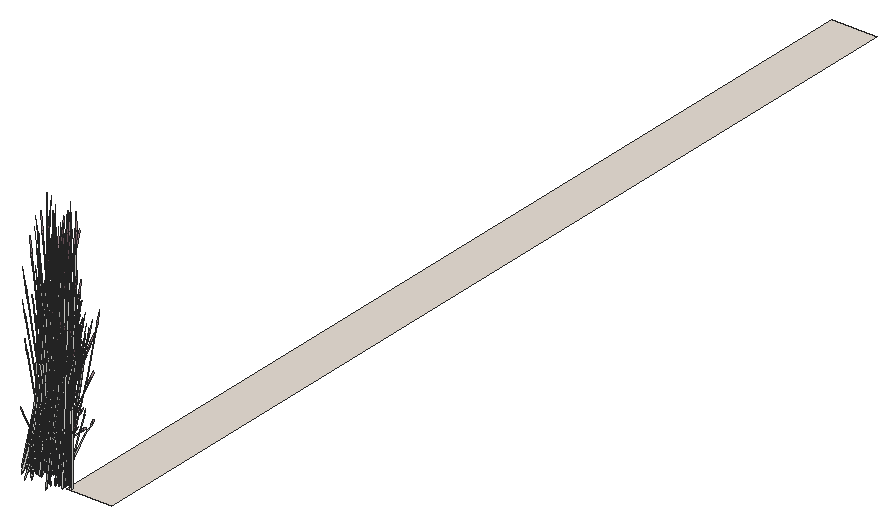
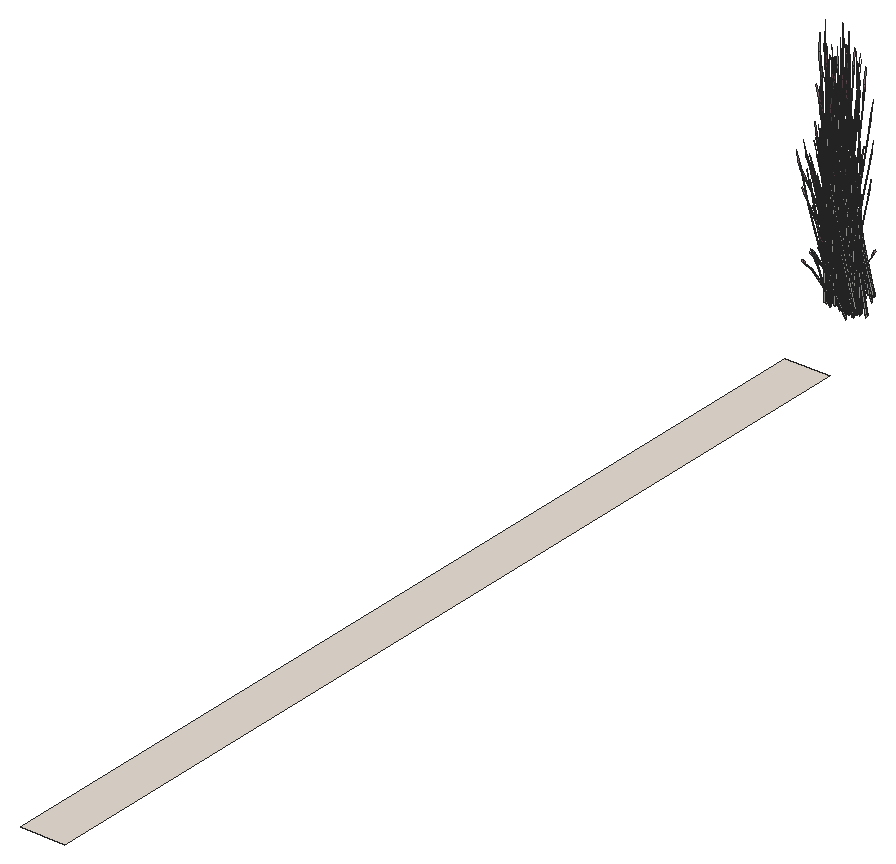
# SketchUp Ruby script. Lengths in inches.
U = 1.inch
M = Sketchup.active_model
def pt(a) = Geom::Point3d.new(a.map { |v| v * U })
def face(e, loops, mat)
  f = e.add_face(loops[0].map { |a| pt(a) })
  loops[1..].each { |l| e.add_face(l.map { |a| pt(a) }).erase! }
  f.material = f.back_material = mat if mat
  f
end
# faces: each face lists its corners as indices into pts; further lists are holes
def faces(e, pts, list, mat = nil) = list.each { |f| face(e, (f[0].is_a?(Array) ? f : [f]).map { |l| l.map { |i| pts[i] } }, mat) }
# xy, xz, yz: faces in a plane at the given z, y or x. An outline is a flat list of corners, or four numbers for a rectangle; further outlines are holes
def ring(l) = l.size == 4 ? [[l[0], l[1]], [l[2], l[1]], [l[2], l[3]], [l[0], l[3]]] : l.each_slice(2).to_a
def flat(e, list, mat, &to3) = list.each { |f| face(e, (f[0].is_a?(Array) ? f : [f]).map { |l| ring(l).map { |u, v| to3.(u, v) } }, mat) }
def xy(e, z, list, mat = nil) = flat(e, list, mat) { |x, y| [x, y, z] }
def xz(e, y, list, mat = nil) = flat(e, list, mat) { |x, z| [x, y, z] }
def yz(e, x, list, mat = nil) = flat(e, list, mat) { |y, z| [x, y, z] }
def lines(e, pts, list) = list.each { |a, b| e.add_line(pt(pts[a]), pt(pts[b])) }
# prism: a flat outline (further loops are holes) pulled along v
def prism(e, loops, v, mat = nil)
  f = face(e, loops, mat); d = Geom::Vector3d.new(v.map { |x| x * U })
  f.pushpull(f.normal.samedirection?(d) ? d.length : -d.length)
end
def box(e, o, s, mat = nil) = prism(e, [[o, [o[0] + s[0], o[1], o[2]], [o[0] + s[0], o[1] + s[1], o[2]], [o[0], o[1] + s[1], o[2]]]], [0, 0, s[2]], mat)
def at(x, y, z, deg = 0) = Geom::Transformation.translation(pt([x, y, z])) * Geom::Transformation.rotation(ORIGIN, Z_AXIS, deg.degrees)
def axes(o, x, y, z) = Geom::Transformation.new([*x, 0, *y, 0, *z, 0, *pt(o).to_a, 1])
def part(name) = M.definitions.add(name)
# library, detail: a bought-in or finely detailed component or shape, given as its bounding box
def library(name, o, s) = part(name).tap { |d| box(d.entities, o, s) }
def detail(e, o, s) = box(e.add_group.entities, o, s)
def put(e, d, t, mat = nil) = e.add_instance(d, t).tap { |i| i.material = mat if mat }
def group(e, t, mat = nil) = e.add_group.tap { |g| g.transformation = t; g.material = mat if mat }.entities
root = M.entities
M.materials.add("LightPink_Translucent").color = [144, 107, 117]
M.materials["LightPink_Translucent"].alpha = 0.75
M.materials.add("Marble_01_1K").color = [230, 221, 211]
c1 = part("blade")
p = [[2.15,0.21,22],[0,0.17,0],[0.09,0.45,0],[2.18,0.31,22],[2.29,0.31,22],[0.38,0.45,0],
  [2.48,0.24,33],[2.49,0.24,33],[2.48,0.22,33]]
faces(c1.entities,p,[[0,1,2,3],[4,5,2,3],[6,3,4,7],[8,0,3,6]])
c2 = part("seeds")
p = [[0.3,-0.1,1.38],[-0.01,-0.03,1.59],[-0.01,-0.03,0.03],[0.14,-0.07,-0.07],[0.29,-0.03,3],[0.15,0.01,3.11]]
faces(c2.entities,p,[[0,1,2,3],[1,0,4,5]],"LightPink_Translucent")
c3 = part("blade with seeds")
put(c3.entities,c1,at(0,0,0))
put(c3.entities,c2,axes([2.4,0.25,30.99],[1.5799,-0.05474,1.17369],[-0.12525,1.92788,0.29478],[-0.07173,-0.02425,1.56792]))
xy(root,36,[[314,46,324,262]],"Marble_01_1K")
put(root,c3,axes([315.7,32.58,46.14],[0.49824,-0.09289,-0.45151],[0.08716,0.35177,-0.34973],[0.13382,0.10081,0.86392]))
put(root,c3,axes([317.83,36.3125,46.16],[-0.06595,-0.00297,1.56736],[-0.27386,-0.31799,-0.1481],[0.10998,-0.10455,0.27737]))
put(root,c3,axes([320.91,35.45,43.82],[-0.52523,-0.06406,-0.55095],[0.11084,-0.39517,-0.1446],[-0.15674,-0.04788,1.21613]))
put(root,c3,axes([314.6,36.14,43.82],[0.34009,-0.2937,-0.55095],[0.42248,0.26632,-0.1446],[0.13628,-0.07327,1.21613]))
put(root,c3,axes([317.05,35.44,44.44],[-0.16818,0.19891,1.01491],[-0.14456,-0.26725,0.74569],[0.1389,-0.06697,0.22354]))
put(root,c3,axes([321.16,30.84,44.97],[0.01109,-0.20172,1.3638],[0.49896,0.10655,0.18846],[-0.04323,0.21498,0.64398]))
put(root,c3,axes([322.19,35.24,44.03],[-0.46965,-0.33633,-0.05417],[0.46994,-0.33653,0],[-0.0164,-0.01174,1.55135]))
put(root,c3,axes([321.01,34.03,44.1875],[-0.14586,0.38834,0.15589],[-0.53375,-0.1099,0.31002],[0.0922,-0.00189,1.41735]))
put(root,c3,axes([316.39,32.93,44.36],[-0.32378,-0.01225,0.92831],[0.21383,-0.26028,0.51254],[0.12791,0.09247,0.72818]))
put(root,c3,axes([319.27,34.71,46.18],[0.14265,-0.35629,0.42415],[0.46898,0.12183,0.34973],[-0.18443,0.02141,0.87768]))
put(root,c3,axes([316.8125,36.1875,46],[0.43951,-0.05584,-0.31292],[0.11606,0.31924,0.40398],[0.12595,-0.08575,0.77298]))
put(root,c3,axes([315.46,32.86,46.18],[-0.22948,0.24822,0.05682],[-0.32679,-0.14452,0.44729],[0.10565,0.07958,0.68204]))
put(root,c3,axes([319.23,34.61,46.18],[-0.18545,-0.26643,0.05682],[0.33817,-0.13041,0.44729],[-0.14907,0.02573,0.68204]))
put(root,c3,axes([321.3,35.29,44.09],[0.63817,0.08233,0.40429],[-0.12987,0.46497,0.15865],[-0.09326,-0.0449,1.40366]))
put(root,c3,axes([314.92,33.7,46.99],[0.34892,-0.22417,-0.05733],[0.3197,0.24551,-0.25992],[0.02251,0.06957,0.85731]))
put(root,c3,axes([315.55,32.79,46.18],[-0.5022,0.08967,0.42415],[-0.08716,-0.35177,0.34973],[0.11811,0.10367,0.87768]))
put(root,c3,axes([319.22,34.89,43.32],[0.0128,0.06158,1.55816],[-0.25814,0.3216,-0.23804],[-0.18336,-0.01621,0.26541]))
put(root,c3,axes([314.23,36.48,44.36],[-0.05884,-0.44587,-0.25709],[0.6128,-0.02696,-0.44182],[0.10791,-0.05939,1.41118]))
put(root,c3,axes([320.35,36.05,43.79],[-0.11861,-0.34048,-0.27372],[0.47106,-0.09668,0.27372],[-0.09497,-0.03926,1.22797]))
put(root,c3,axes([316.46,36.375,46.46],[-0.43951,0.05584,0.31292],[-0.11606,-0.31924,-0.40398],[0.12595,-0.08575,0.77298]))
put(root,c3,axes([315.33,32.3,44.29],[0.00891,-0.12953,1.26356],[0.4258,-0.14469,-0.27174],[0.13144,0.15503,0.54024]))
put(root,c3,axes([320.96,36.03,44.1875],[0.54257,-0.10371,0.15589],[0.13397,0.38597,0.31002],[-0.04839,-0.05624,1.41735]))
put(root,c3,axes([314.15,35.49,43.79],[0.47106,0.09668,-0.27372],[-0.11861,0.34048,0.27372],[0.09497,-0.03926,1.22797]))
put(root,c3,axes([314.17,32.76,46.45],[0.49409,-0.18193,-0.10745],[0.24281,0.32289,-0.59638],[0.06519,0.13607,0.90619]))
put(root,c3,axes([320.22,36.19,43.78],[-0.47255,-0.19538,-0.43871],[0.28245,-0.35034,0],[-0.10763,-0.0445,1.3917]))
put(root,c3,axes([321.51,35.51,44.36],[-0.50979,0.25942,-0.25709],[-0.339,-0.36656,-0.44182],[-0.12578,-0.03723,1.41118]))
put(root,c3,axes([322.625,34.05,44.1875],[-0.54257,0.10371,0.15589],[-0.13397,-0.38597,0.31002],[0.04839,0.05624,1.41735]))
put(root,c3,axes([316.85,36.33,46.18],[0.34663,0.16434,0.05682],[-0.20181,0.23402,0.44729],[0.11113,-0.07566,0.68204]))
put(root,c3,axes([316.76,36.26,46.18],[0.12522,0.35963,0.42415],[-0.49122,0.06241,0.34973],[0.14477,-0.08458,0.87768]))
put(root,c3,axes([318.08,36.69,46.17],[0.07006,-0.05952,1.54581],[-0.08968,-0.3651,-0.24447],[0.1758,-0.06922,0.12397]))
put(root,c3,axes([314.6,32.74,46.14],[0.49634,0.09796,-0.45151],[-0.17013,0.33585,-0.34973],[0.04551,0.13522,0.86392]))
put(root,c3,axes([314.88,32.05,45.43],[-0.11542,-0.12546,1.51428],[0.53333,-0.10562,0.12244],[0.12054,0.19696,0.64734]))
put(root,c3,axes([321.77,35.9375,43.95],[-0.16474,-0.33688,0],[0.47043,-0.11798,0],[0,0,1.36402]))
put(root,c3,axes([321.46,35.62,44.3125],[-0.09741,0.34873,0.12794],[-0.4759,-0.06053,-0.36534],[-0.08661,-0.03581,1.11991]))
put(root,c3,axes([319.61,34.71,46.46],[0.41962,0.10901,0.31292],[-0.12239,0.31802,-0.40398],[-0.16894,0.02916,0.77298]))
put(root,c3,axes([322.57,36.05,44.1875],[0.14586,-0.38834,0.15589],[0.53375,0.1099,0.31002],[-0.0922,0.00189,1.41735]))
put(root,c3,axes([323.41,35.06,44.1875],[-0.39671,-0.28463,0.15589],[0.39978,-0.27607,0.31002],[-0.04381,0.05813,1.41735]))
put(root,c3,axes([321.66,36.09,43.94],[-0.50902,-0.17543,0],[0.24498,-0.36452,0],[0,0,1.43768]))
put(root,c3,axes([322.08,35.625,44.18],[-0.49304,-0.31451,-0.2226],[0.41487,-0.35316,0.48713],[-0.13277,0.03679,1.48635]))
put(root,c3,axes([320.78,36.23,44.19],[0.47255,0.19538,0.43871],[-0.28245,0.35034,0],[-0.10763,-0.0445,1.3917]))
put(root,c3,axes([316.7,37.25,46.45],[-0.25405,-0.35383,-0.10745],[0.45089,-0.17388,-0.59638],[0.19001,-0.04668,0.90619]))
put(root,c3,axes([316.68,36.94,46.14],[0.13679,-0.35544,-0.45151],[0.46898,0.12183,-0.34973],[0.18882,-0.03259,0.86392]))
put(root,c3,axes([315.9375,35.5,44.1],[0.31568,-0.39156,0],[0.52815,0.21836,-0.456],[0.12029,0.04973,1.44655]))
put(root,c3,axes([322.35,35.08,44.03],[0,0.45191,-0.04981],[-0.63136,0,0],[0,0.0142,1.58489]))
put(root,c3,axes([319.43,34.61,46.45],[0.25405,0.35383,-0.10745],[-0.45089,0.17388,-0.59638],[-0.19001,0.04668,0.90619]))
put(root,c3,axes([317.18,37.04,43.75],[-0.3252,0.04689,1.25103],[-0.05176,-0.37326,0.07161],[0.22777,-0.0565,0.71188]))
put(root,c3,axes([317.77,36.71,44],[-0.31304,-0.24986,-0.05733],[0.34284,-0.22894,-0.25992],[0.09714,-0.01612,0.85731]))
put(root,c3,axes([320.51,36.43,44.1],[-0.31568,0.39156,0],[-0.52815,-0.21836,-0.456],[-0.12029,-0.04973,1.44655]))
put(root,c3,axes([322.32,35.36,44.4],[0.54829,-0.02412,0.39531],[0.04958,0.40041,-0.19025],[-0.09816,0.04058,1.26923]))
put(root,c3,axes([315.67,35.7,44.19],[-0.47255,-0.19538,0.43871],[0.28245,-0.35034,0],[0.10763,0.0445,1.3917]))
put(root,c3,axes([316.59,37.07,46.4],[0.44368,-0.17257,-0.62776],[0.24726,0.35524,0.07576],[0.21437,-0.04035,0.88802]))
put(root,c3,axes([321.83,35.56,43.95],[-0.54829,0.02412,-0.39531],[-0.04958,-0.40041,0.19025],[-0.09816,0.04058,1.26923]))
put(root,c3,axes([316.52,37.14,46.46],[-0.41962,-0.10901,0.31292],[0.12239,-0.31802,-0.40398],[0.16894,-0.02916,0.77298]))
put(root,c3,axes([313.65,36.1875,43.41],[-0.49699,0.15644,1.13921],[-0.15819,-0.44887,0.44265],[0.30518,0.00747,1.29573]))
put(root,c3,axes([314.99,36.31,44.3125],[0.09741,-0.34873,0.12794],[0.4759,0.06053,-0.36534],[0.08661,0.03581,1.11991]))
put(root,c3,axes([322.4375,36.48,43.9375],[-0.31175,-0.39292,-0.04544],[0.52815,-0.21836,0.456],[-0.13015,0.03741,1.44584]))
put(root,c3,axes([317.54,36.8,43.32],[-0.02639,-0.05932,1.55816],[0.18302,-0.34702,-0.23804],[0.18462,-0.00499,0.26541]))
put(root,c3,axes([322.33,35.53,44.3125],[0.37303,0.23477,0.12794],[-0.31115,0.26487,-0.36534],[-0.08661,0.03581,1.11991]))
put(root,c3,axes([319.38,35.6,46.18],[-0.12522,-0.35963,0.42415],[0.49122,-0.06241,0.34973],[-0.14477,0.08458,0.87768]))
put(root,c3,axes([319.28,35.53,46.18],[-0.34663,-0.16434,0.05682],[0.20181,-0.23402,0.44729],[-0.11113,0.07566,0.68204]))
put(root,c3,axes([314.79,36.4,44.4],[-0.30332,-0.32798,0.39531],[0.45944,-0.23096,-0.19025],[0.09816,0.04058,1.26923]))
put(root,c3,axes([314.94,36.42,44.36],[0.50979,-0.25942,-0.25709],[0.339,0.36656,-0.44182],[0.12578,0.03723,1.41118]))
put(root,c3,axes([316.97,37.1,46],[0.41962,0.10901,-0.31292],[-0.12239,0.31802,0.40398],[0.16894,-0.02916,0.77298]))
put(root,c3,axes([322.72,36.26,44.19],[0.47255,-0.19538,0.43871],[0.28245,0.35034,0],[-0.10763,0.0445,1.3917]))
put(root,c3,axes([316.23,35.73,43.78],[0.47255,0.19538,-0.43871],[-0.28245,0.35034,0],[0.10763,0.0445,1.3917]))
put(root,c3,axes([322.05,35.95,44.02],[0.21952,0.44891,-0.05313],[-0.62724,0.1573,0],[0.00767,0.01568,1.52132]))
put(root,c3,axes([315.33,36.85,43.95],[0.56491,0,0],[0,0.40454,0],[0,0,1.5764]))
put(root,c3,axes([322.29,36.44,43.79],[-0.47106,-0.09668,-0.27372],[0.11861,-0.34048,0.27372],[-0.09497,0.03926,1.22797]))
put(root,c3,axes([319.68,35.48,46.46],[0.43951,-0.05584,0.31292],[0.11606,0.31924,-0.40398],[-0.12595,0.08575,0.77298]))
put(root,c3,axes([323.86,35.36,43.94],[-0.63105,-0.00312,-0.04397],[0,-0.43672,0.44129],[-0.01983,0.09942,1.3992]))
put(root,c3,axes([315.82,36.71,45.43],[-0.20943,0.00885,1.51428],[0.13893,-0.38357,0.12244],[0.29846,0.02372,0.64734]))
put(root,c3,axes([316.09,35.875,43.79],[0.11861,0.34048,-0.27372],[-0.47106,0.09668,0.27372],[0.09497,0.03926,1.22797]))
put(root,c3,axes([318.53,36.43,44.44],[0.21042,-0.1771,1.01491],[0.08303,0.28036,0.74569],[-0.15207,0.0502,0.22354]))
put(root,c3,axes([322.21,35.45,44.36],[0.05884,0.44587,-0.25709],[-0.6128,0.02696,-0.44182],[-0.10791,0.05939,1.41118]))
put(root,c3,axes([316.91,37.24,46.18],[0.18545,0.26643,0.05682],[-0.33817,0.13041,0.44729],[0.14907,-0.02573,0.68204]))
put(root,c3,axes([322.4375,35.27,43.95],[-0.24498,0.3521,-0.39531],[-0.50902,-0.16945,0.19025],[0,0.08116,1.26923]))
put(root,c3,axes([319.32,35.67,46],[-0.43951,0.05584,-0.31292],[-0.11606,-0.31924,0.40398],[-0.12595,0.08575,0.77298]))
put(root,c3,axes([315.15,36.64,44.1],[-0.63817,-0.08233,0.43472],[0.12987,-0.46497,0.17059],[0.09326,0.0449,1.50931]))
put(root,c3,axes([316.87,37.14,46.18],[-0.14265,0.35629,0.42415],[-0.46898,-0.12183,0.34973],[0.18443,-0.02141,0.87768]))
put(root,c3,axes([315.25,37.74,43.93],[0.53009,-0.13258,-0.16963],[0.18627,0.38191,0.00007],[0.05851,-0.01465,1.53656]))
put(root,c3,axes([318.68,36.38,46.99],[0.44556,0.1043,-0.05733],[-0.13706,0.32103,-0.25992],[-0.07288,0.04874,0.85731]))
put(root,c3,axes([321.84,35.79,43.82],[-0.34009,0.2937,-0.55095],[-0.42248,-0.26632,-0.1446],[-0.13628,0.07327,1.21613]))
put(root,c3,axes([315.54,36.48,43.82],[0.52523,0.06406,-0.55095],[-0.11084,0.39517,-0.1446],[0.15674,0.04788,1.21613]))
put(root,c3,axes([317.86,37.17,44.44],[-0.31197,0.06451,1.01491],[0.14684,-0.26661,0.74569],[0.1655,0.01824,0.22354]))
put(root,c3,axes([322.45,36.28,44.06],[0.63212,0.12701,0.27176],[-0.15814,0.45398,-0.32244],[-0.10462,0.05682,1.45692]))
put(root,c3,axes([322.4,36.59,43.78],[-0.47255,0.19538,-0.43871],[-0.28245,-0.35034,0],[-0.10763,0.0445,1.3917]))
put(root,c3,axes([317.71,38.3,46.16],[-0.04566,-0.03421,1.56736],[0.09987,-0.36669,-0.1481],[0.17984,-0.02343,0.27737]))
put(root,c3,axes([319.45,35.45,46.45],[0.46706,0.21546,-0.10745],[-0.26908,0.31203,-0.59638],[-0.13196,0.10846,0.90619]))
put(root,c3,axes([315.26,36.6,43.95],[0.30332,0.32798,-0.39531],[-0.45944,0.23096,0.19025],[0.09816,0.04058,1.26923]))
put(root,c3,axes([317.32,37.99,45.47],[-0.09664,-0.32847,-0.03085],[0.45676,-0.07551,-0.13989],[0.09538,0.02082,0.4614]))
put(root,c3,axes([316.13,37.98,46.45],[0.02704,-0.39739,-0.10745],[0.51189,0.01086,-0.59638],[0.19715,0.0276,0.90619]))
put(root,c3,axes([320.08,35.35,45.43],[0.12611,-0.12006,1.51428],[0.31843,0.32408,0.12244],[-0.2184,0.14759,0.64734]))
put(root,c3,axes([319.69,35.7,46.14],[0.12971,0.3568,-0.45151],[-0.49122,0.06241,-0.34973],[-0.14077,0.09583,0.86392]))
put(root,c3,axes([316.6,36.92,44.19],[0,-0.39075,0.43871],[0.56491,0,0],[0,0.089,1.3917]))
put(root,c3,axes([315.52,36.8,44.3125],[0.47043,-0.11396,0.12794],[0.16474,0.32541,-0.36534],[0,0.07162,1.11991]))
put(root,c3,axes([320.27,36.11,46.46],[0.34164,-0.20573,0.31292],[0.3234,0.23491,-0.40398],[-0.04921,0.11936,0.77298]))
put(root,c3,axes([322.83,36.53,44.1],[0.31568,0.39156,0],[-0.52815,0.21836,-0.456],[-0.12029,0.04973,1.44655]))
put(root,c3,axes([316.05,37.83,46.46],[-0.28729,-0.24465,0.31292],[0.32804,-0.23159,-0.40398],[0.16667,0.03524,0.77298]))
put(root,c3,axes([322.56,34.98,44.51],[-0.01379,-0.36791,1.24828],[0.62424,0.09537,0.52853],[-0.14764,0.20132,1.17828]))
put(root,c3,axes([319.97,36.3,46.18],[-0.41493,-0.01821,0.05682],[0.01138,-0.27493,0.44729],[-0.04342,0.10531,0.68204]))
put(root,c3,axes([319.08,36.61,43.32],[0.06773,0.03904,1.55816],[0.11484,0.36171,-0.23804],[-0.15011,0.07713,0.26541]))
put(root,c3,axes([320.1,36.32,46.18],[-0.35954,-0.26661,0.42415],[0.38183,-0.22994,0.34973],[-0.06632,0.12508,0.87768]))
put(root,c3,axes([317.27,37.6,44.29],[-0.1216,-0.0961,1.26356],[0.15822,-0.31792,-0.27174],[0.24603,0.04307,0.54024]))
put(root,c3,axes([321.23,36.45,46.46],[0.15222,-0.30049,0.31292],[0.44409,0.08764,-0.40398],[0.04072,0.12098,0.77298]))
put(root,c3,axes([316.58,37.74,46.17],[0.10831,-0.00661,1.54581],[0.29709,-0.30358,-0.24447],[0.19266,0.04007,0.12397]))
put(root,c3,axes([316.16,37.79,46.4],[0.50473,0.00941,-0.62776],[-0.0339,0.39618,0.07576],[0.21383,0.04181,0.88802]))
put(root,c3,axes([319.99,35.65,45.43],[0.09401,-0.13431,1.51428],[0.3944,0.27795,0.12244],[-0.17792,0.17323,0.64734]))
put(root,c3,axes([321.09,36.72,46.18],[-0.37205,0.1328,0.05682],[-0.18211,-0.24217,0.44729],[0.03593,0.10675,0.68204]))
put(root,c3,axes([320.1,36.4,46],[-0.34164,0.20573,-0.31292],[-0.3234,-0.23491,0.40398],[-0.04921,0.11936,0.77298]))
put(root,c3,axes([318.92,36.34,46.17],[-0.01255,0.07733,1.54581],[0.35618,0.269,-0.24447],[-0.09325,0.12721,0.12397]))
put(root,c3,axes([320.06,36.17,46.77],[0.55492,0.01936,-0.11927],[-0.01517,0.36657,-0.66198],[-0.03855,0.14118,1.00587]))
put(root,c3,axes([321.23,36.7,46.47],[-0.49753,-0.10215,0.47081],[0.17013,-0.33585,0.3882],[0.0299,0.13207,0.97422]))
put(root,c3,axes([316.98,36.99,44.1],[0.63136,0,0],[0,0.43672,-0.456],[0,0.09947,1.44655]))
put(root,c3,axes([320.3125,37.2,44.44],[-0.01307,-0.23234,1.01491],[0.32652,0.16572,0.74569],[-0.06422,0.11074,0.22354]))
put(root,c3,axes([315.36,36.83,44.36],[0.56863,0.18645,-0.25709],[-0.2738,0.39352,-0.44182],[0.01787,0.09662,1.41118]))
put(root,c3,axes([316.46,37.95,46],[0.28729,0.24465,-0.31292],[-0.32804,0.23159,0.40398],[0.16667,0.03524,0.77298]))
put(root,c3,axes([316.6,37.27,43.79],[-0.35245,0.2438,-0.27372],[-0.35245,-0.2438,0.27372],[0,0.07853,1.22797]))
put(root,c3,axes([321.17,36.65,43.32],[0.08172,-0.02126,1.55816],[0.49154,0.11703,-0.23804],[0.01437,0.1319,0.26541]))
put(root,c3,axes([316.3125,38.05,46.18],[-0.02542,0.29714,0.05682],[-0.38391,-0.00815,0.44729],[0.14706,0.03109,0.68204]))
put(root,c3,axes([316.35,37.95,46.18],[-0.3723,0.25748,0.42415],[-0.32109,-0.27343,0.34973],[0.17467,0.04749,0.87768]))
put(root,c3,axes([320.4375,36.31,46.42],[0.36145,0.26255,-0.50118],[-0.38183,0.22994,-0.3882],[-0.055,0.1334,0.95895]))
put(root,c3,axes([320.04,36.7,44.49],[0.45869,-0.0692,0.0575],[0.10545,0.27878,-0.76259],[-0.02908,0.14112,0.68355]))
put(root,c3,axes([321.28,36.77,46],[-0.15222,0.30049,-0.31292],[-0.44409,-0.08764,0.40398],[0.04072,0.12098,0.77298]))
put(root,c3,axes([315.16,38.25,46.46],[-0.07798,-0.31474,0.31292],[0.44579,-0.08311,-0.40398],[0.11974,0.09019,0.77298]))
put(root,c3,axes([316.84,37.28,43.78],[0,0.39075,-0.43871],[-0.56491,0,0],[0,0.089,1.3917]))
put(root,c3,axes([320.32,36.1875,46.72],[-0.01314,0.36145,-0.69681],[-0.55324,-0.02428,0.08409],[-0.05838,0.15313,0.9857]))
put(root,c3,axes([315.43,37.33,45.43],[-0.18755,-0.06732,1.51428],[0.38813,-0.28243,0.12244],[0.24191,0.12741,0.64734]))
put(root,c3,axes([318.88,37.14,46.16],[0.05728,-0.02359,1.56736],[0.47345,0.15692,-0.1481],[-0.01113,0.13066,0.27737]))
put(root,c3,axes([315.46,36.44,45.95],[-0.4363,-0.20303,1.22187],[0.46069,-0.31611,0.5272],[0.14077,0.1905,1.18105]))
put(root,c3,axes([320.85,35.93,45.43],[-0.01236,-0.14998,1.51428],[0.53562,0.09949,0.12244],[-0.03313,0.21373,0.64734]))
put(root,c3,axes([316.12,38.09,44.44],[-0.28429,-0.11236,1.01491],[0.36709,-0.11416,0.74569],[0.09901,0.0967,0.22354]))
put(root,c3,axes([315.125,38.41,46.45],[0.30087,-0.33447,-0.10745],[0.43572,0.19269,-0.59638],[0.15146,0.0945,0.90619]))
put(root,c3,axes([321.33,36.5,46.4],[0.24099,0.31773,-0.62776],[-0.49607,0.17707,0.07576],[0.05635,0.15352,0.88802]))
put(root,c3,axes([319.93,37,44.29],[0.15933,-0.06164,1.26356],[0.39339,0.18587,-0.27174],[-0.11709,0.16083,0.54024]))
put(root,c3,axes([320.97,37.3,46.17],[0.064,0.06292,1.54581],[0.51651,0.02472,-0.24447],[0.05194,0.13877,0.12397]))
put(root,c3,axes([314.73,38.69,46.16],[0.00149,-0.04731,1.56736],[0.4327,-0.20872,-0.1481],[0.1503,0.0745,0.27737]))
put(root,c3,axes([316.2,38.51,43.32],[0.03679,-0.05641,1.55816],[0.46313,-0.16615,-0.23804],[0.14041,0.08599,0.26541]))
put(root,c3,axes([315.59,37.23,43.85],[0.18514,0.35777,-0.61156],[-0.53331,0.12885,-0.16051],[0.02046,0.12115,1.3499]))
put(root,c3,axes([315.48,38.25,46.14],[0.49824,-0.09289,-0.45151],[0.08716,0.35177,-0.34973],[0.13382,0.10081,0.86392]))
put(root,c3,axes([316.17,38.6,44.36],[-0.32378,-0.01225,0.92831],[0.21383,-0.26028,0.51254],[0.12791,0.09247,0.72818]))
put(root,c3,axes([315.23,38.54,46.18],[-0.22948,0.24822,0.05682],[-0.32679,-0.14452,0.44729],[0.10565,0.07958,0.68204]))
put(root,c3,axes([320.14,36.7,44.97],[0.01109,-0.20172,1.3638],[0.49896,0.10655,0.18846],[-0.04323,0.21498,0.64398]))
put(root,c3,axes([315.33,38.47,46.18],[-0.5022,0.08967,0.42415],[-0.08716,-0.35177,0.34973],[0.11811,0.10367,0.87768]))
put(root,c3,axes([315.11,37.97,44.29],[0.00891,-0.12953,1.26356],[0.4258,-0.14469,-0.27174],[0.13144,0.15503,0.54024]))
put(root,c3,axes([313.95,38.43,46.45],[0.49409,-0.18193,-0.10745],[0.24281,0.32289,-0.59638],[0.06519,0.13607,0.90619]))
put(root,c3,axes([314.375,38.41,46.14],[0.49634,0.09796,-0.45151],[-0.17013,0.33585,-0.34973],[0.04551,0.13522,0.86392]))
put(root,c3,axes([314.66,37.72,45.43],[-0.11542,-0.12546,1.51428],[0.53333,-0.10562,0.12244],[0.12054,0.19696,0.64734]))
